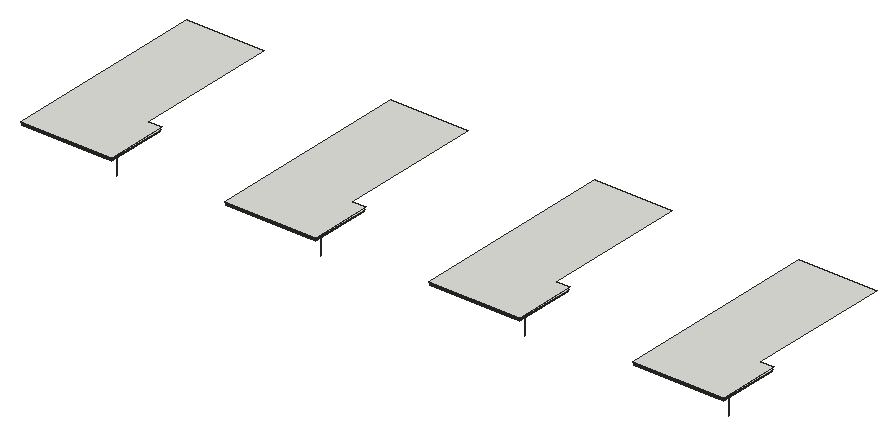
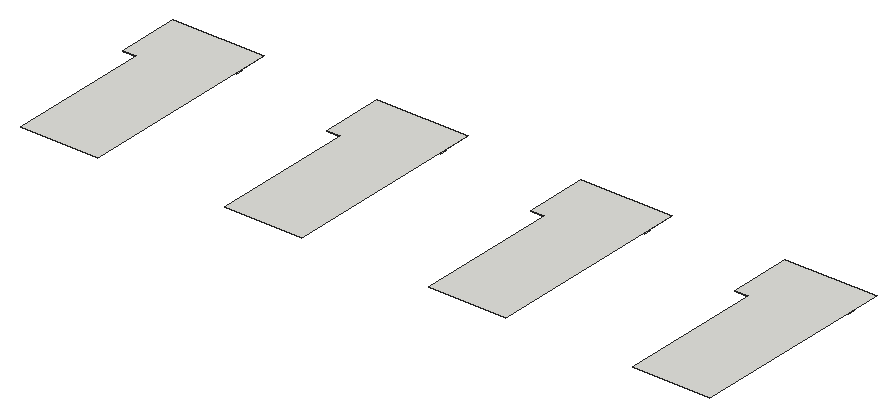
# SketchUp Ruby script. Lengths in inches.
U = 1.inch
M = Sketchup.active_model
def pt(a) = Geom::Point3d.new(a.map { |v| v * U })
def face(e, loops, mat)
  f = e.add_face(loops[0].map { |a| pt(a) })
  loops[1..].each { |l| e.add_face(l.map { |a| pt(a) }).erase! }
  f.material = f.back_material = mat if mat
  f
end
# faces: each face lists its corners as indices into pts; further lists are holes
def faces(e, pts, list, mat = nil) = list.each { |f| face(e, (f[0].is_a?(Array) ? f : [f]).map { |l| l.map { |i| pts[i] } }, mat) }
# xy, xz, yz: faces in a plane at the given z, y or x. An outline is a flat list of corners, or four numbers for a rectangle; further outlines are holes
def ring(l) = l.size == 4 ? [[l[0], l[1]], [l[2], l[1]], [l[2], l[3]], [l[0], l[3]]] : l.each_slice(2).to_a
def flat(e, list, mat, &to3) = list.each { |f| face(e, (f[0].is_a?(Array) ? f : [f]).map { |l| ring(l).map { |u, v| to3.(u, v) } }, mat) }
def xy(e, z, list, mat = nil) = flat(e, list, mat) { |x, y| [x, y, z] }
def xz(e, y, list, mat = nil) = flat(e, list, mat) { |x, z| [x, y, z] }
def yz(e, x, list, mat = nil) = flat(e, list, mat) { |y, z| [x, y, z] }
def lines(e, pts, list) = list.each { |a, b| e.add_line(pt(pts[a]), pt(pts[b])) }
# prism: a flat outline (further loops are holes) pulled along v
def prism(e, loops, v, mat = nil)
  f = face(e, loops, mat); d = Geom::Vector3d.new(v.map { |x| x * U })
  f.pushpull(f.normal.samedirection?(d) ? d.length : -d.length)
end
def box(e, o, s, mat = nil) = prism(e, [[o, [o[0] + s[0], o[1], o[2]], [o[0] + s[0], o[1] + s[1], o[2]], [o[0], o[1] + s[1], o[2]]]], [0, 0, s[2]], mat)
def at(x, y, z, deg = 0) = Geom::Transformation.translation(pt([x, y, z])) * Geom::Transformation.rotation(ORIGIN, Z_AXIS, deg.degrees)
def axes(o, x, y, z) = Geom::Transformation.new([*x, 0, *y, 0, *z, 0, *pt(o).to_a, 1])
def part(name) = M.definitions.add(name)
# library, detail: a bought-in or finely detailed component or shape, given as its bounding box
def library(name, o, s) = part(name).tap { |d| box(d.entities, o, s) }
def detail(e, o, s) = box(e.add_group.entities, o, s)
def put(e, d, t, mat = nil) = e.add_instance(d, t).tap { |i| i.material = mat if mat }
def group(e, t, mat = nil) = e.add_group.tap { |g| g.transformation = t; g.material = mat if mat }.entities
root = M.entities
M.materials.add("[0136_Charcoal]").color = [35, 35, 35]
M.materials.add("[Color M09]").color = [0, 0, 0]
M.materials.add("[Translucent Glass Gray]").color = [128, 128, 128]
M.materials["[Translucent Glass Gray]"].alpha = 0.5
xy(root,225.74,[[410.54,519.01,443.7,522.83],[1000.35,519.01,1033.52,522.83],[1590.16,519.01,1623.33,522.83],[2179.98,519.01,2213.14,522.83]])
xy(root,225.74,[[412.04,509.7,443.7,511.7],[445.2,509.7,475.37,511.7],[476.87,509.7,507.04,511.7],[1001.85,509.7,1033.52,511.7],[1035.02,509.7,1065.18,511.7],
  [1066.68,509.7,1096.85,511.7],[1591.66,509.7,1623.33,511.7],[1624.83,509.7,1655,511.7],[1656.5,509.7,1686.66,511.7],[2181.48,509.7,2213.14,511.7],
  [2214.64,509.7,2244.81,511.7],[2246.31,509.7,2276.48,511.7],[515.04,521.34,518.04,553.96],[1104.85,521.34,1107.85,553.96],[1694.66,521.34,1697.66,553.96],
  [2284.48,521.34,2287.48,553.96],[515.04,555.96,518.04,586.08],[1104.85,555.96,1107.85,586.08],[1694.66,555.96,1697.66,586.08],[2284.48,555.96,2287.48,586.08],
  [515.04,588.08,518.04,619.7],[1104.85,588.08,1107.85,619.7],[1694.66,588.08,1697.66,619.7],[2284.48,588.08,2287.48,619.7]],"[Color M09]")
xy(root,227.74,[[412.04,509.7,443.7,511.7],[445.2,509.7,475.37,511.7],[476.87,509.7,507.04,511.7],[1001.85,509.7,1033.52,511.7],[1035.02,509.7,1065.18,511.7],
  [1066.68,509.7,1096.85,511.7],[1591.66,509.7,1623.33,511.7],[1624.83,509.7,1655,511.7],[1656.5,509.7,1686.66,511.7],[2181.48,509.7,2213.14,511.7],
  [2214.64,509.7,2244.81,511.7],[2246.31,509.7,2276.48,511.7],[515.04,521.34,518.04,553.96],[1104.85,521.34,1107.85,553.96],[1694.66,521.34,1697.66,553.96],
  [2284.48,521.34,2287.48,553.96],[515.04,555.96,518.04,586.08],[1104.85,555.96,1107.85,586.08],[1694.66,555.96,1697.66,586.08],[2284.48,555.96,2287.48,586.08],
  [515.04,588.08,518.04,619.7],[1104.85,588.08,1107.85,619.7],[1694.66,588.08,1697.66,619.7],[2284.48,588.08,2287.48,619.7]],"[Color M09]")
xy(root,240.6,[[311.04,509.7,359.04,525.45],[900.85,509.7,948.85,525.45],[1490.66,509.7,1538.66,525.45],[2080.48,509.7,2128.48,525.45]])
xy(root,249.6875,[[443.7,509.7,445.2,511.7],[475.37,509.7,476.87,511.7],[1033.52,509.7,1035.02,511.7],[1065.18,509.7,1066.68,511.7],[1623.33,509.7,1624.83,511.7],
  [1655,509.7,1656.5,511.7],[2213.14,509.7,2214.64,511.7],[2244.81,509.7,2246.31,511.7],[410.54,511.7,443.7,522.83],[443.7,511.7,476.87,522.83],
  [476.87,511.7,508.54,519.01],[1000.35,511.7,1033.52,522.83],[1033.52,511.7,1066.68,522.83],[1066.68,511.7,1098.35,519.01],[1590.16,511.7,1623.33,522.83],
  [1623.33,511.7,1656.5,522.83],[1656.5,511.7,1688.16,519.01],[2179.98,511.7,2213.14,522.83],[2213.14,511.7,2246.31,522.83],[2246.31,511.7,2277.98,519.01]])
xy(root,249.6875,[[412.04,509.7,443.7,511.7],[445.2,509.7,475.37,511.7],[476.87,509.7,507.04,511.7],[1001.85,509.7,1033.52,511.7],[1035.02,509.7,1065.18,511.7],
  [1066.68,509.7,1096.85,511.7],[1591.66,509.7,1623.33,511.7],[1624.83,509.7,1655,511.7],[1656.5,509.7,1686.66,511.7],[2181.48,509.7,2213.14,511.7],
  [2214.64,509.7,2244.81,511.7],[2246.31,509.7,2276.48,511.7],[515.04,521.34,518.04,553.96],[1104.85,521.34,1107.85,553.96],[1694.66,521.34,1697.66,553.96],
  [2284.48,521.34,2287.48,553.96],[515.04,555.96,518.04,586.08],[1104.85,555.96,1107.85,586.08],[1694.66,555.96,1697.66,586.08],[2284.48,555.96,2287.48,586.08],
  [515.04,588.08,518.04,619.7],[1104.85,588.08,1107.85,619.7],[1694.66,588.08,1697.66,619.7],[2284.48,588.08,2287.48,619.7]],"[Color M09]")
xy(root,251.6875,[[544.21,449.7,557.59,468.65],[1134.02,449.7,1147.4,468.65],[1723.83,449.7,1737.22,468.65],[2313.65,449.7,2327.03,468.65],[410.04,509.7,509.04,511.7],
  [999.85,509.7,1098.85,511.7],[1589.66,509.7,1688.66,511.7],[2179.48,509.7,2278.48,511.7],[503.73,519.34,515.04,555.96],[515.04,519.34,518.04,621.7],
  [1093.54,519.34,1104.85,555.96],[1104.85,519.34,1107.85,621.7],[1683.35,519.34,1694.66,555.96],[1694.66,519.34,1697.66,621.7],[2273.16,519.34,2284.48,555.96],
  [2284.48,519.34,2287.48,621.7],[503.73,555.96,515.04,588.08],[1093.54,555.96,1104.85,588.08],[1683.35,555.96,1694.66,588.08],[2273.16,555.96,2284.48,588.08],
  [503.73,588.08,515.04,621.7],[1093.54,588.08,1104.85,621.7],[1683.35,588.08,1694.66,621.7],[2273.16,588.08,2284.48,621.7]])
xy(root,251.6875,[[302.04,449.7,544.21,509.7],[891.85,449.7,1134.02,509.7],[1481.66,449.7,1723.83,509.7],[2071.48,449.7,2313.65,509.7],[544.21,468.65,544.21,509.7,518.04,509.7,518.04,621.7,557.59,621.7,557.59,468.65],
  [1134.02,468.65,1134.02,509.7,1107.85,509.7,1107.85,621.7,1147.4,621.7,1147.4,468.65],[1723.83,468.65,1723.83,509.7,1697.66,509.7,1697.66,621.7,1737.22,621.7,1737.22,468.65],[2313.65,468.65,2313.65,509.7,2287.48,509.7,2287.48,621.7,2327.03,621.7,2327.03,468.65]],"[0136_Charcoal]")
xy(root,255.07,[[297.83,449.7,557.59,450.7],[887.64,449.7,1147.4,450.7],[1477.46,449.7,1737.22,450.7],[2067.27,449.7,2327.03,450.7],[556.59,450.7,557.59,624.51],
  [1146.4,450.7,1147.4,624.51],[1736.22,450.7,1737.22,624.51],[2326.03,450.7,2327.03,624.51]],"[0136_Charcoal]")
xy(root,256.21,[[296.69,449.7,557.59,450.7],[886.5,449.7,1147.4,450.7],[1476.32,449.7,1737.22,450.7],[2066.13,449.7,2327.03,450.7],[556.59,450.7,557.59,625.64],
  [1146.4,450.7,1147.4,625.64],[1736.22,450.7,1737.22,625.64],[2326.03,450.7,2327.03,625.64]])
xy(root,259.6875,[[293.22,449.7,557.59,449.7,557.59,629.7,518.04,629.7,518.04,1049.7,293.22,1049.7],[883.03,449.7,1147.4,449.7,1147.4,629.7,1107.85,629.7,1107.85,1049.7,883.03,1049.7],[1472.84,449.7,1737.22,449.7,1737.22,629.7,1697.66,629.7,1697.66,1049.7,1472.84,1049.7],[2062.65,449.7,2327.03,449.7,2327.03,629.7,2287.48,629.7,2287.48,1049.7,2062.65,1049.7]])
xz(root,510.7,[[412.04,227.74,443.7,249.6875],[445.2,227.74,475.37,249.6875],[476.87,227.74,507.04,249.6875],[1001.85,227.74,1033.52,249.6875],[1035.02,227.74,1065.18,249.6875],
  [1066.68,227.74,1096.85,249.6875],[1591.66,227.74,1623.33,249.6875],[1624.83,227.74,1655,249.6875],[1656.5,227.74,1686.66,249.6875],[2181.48,227.74,2213.14,249.6875],
  [2214.64,227.74,2244.81,249.6875],[2246.31,227.74,2276.48,249.6875]],"[Translucent Glass Gray]")
xz(root,511.7,[[412.04,225.74,443.7,227.74],[445.2,225.74,475.37,227.61],[476.87,225.74,507.04,227.74],[507.04,225.74,508.54,249.6875],[1001.85,225.74,1033.52,227.74],
  [1035.02,225.74,1065.18,227.61],[1066.68,225.74,1096.85,227.74],[1096.85,225.74,1098.35,249.6875],[1591.66,225.74,1623.33,227.74],[1624.83,225.74,1655,227.61],
  [1656.5,225.74,1686.66,227.74],[1686.66,225.74,1688.16,249.6875],[2181.48,225.74,2213.14,227.74],[2214.64,225.74,2244.81,227.61],[2246.31,225.74,2276.48,227.74],
  [2276.48,225.74,2277.98,249.6875],[410.54,227.74,412.04,249.6875],[443.7,227.74,445.2,231.3],[475.37,227.74,476.87,249.6875],[1000.35,227.74,1001.85,249.6875],
  [1033.52,227.74,1035.02,231.3],[1065.18,227.74,1066.68,249.6875],[1590.16,227.74,1591.66,249.6875],[1623.33,227.74,1624.83,231.3],[1655,227.74,1656.5,249.6875],
  [2179.98,227.74,2181.48,249.6875],[2213.14,227.74,2214.64,231.3],[2244.81,227.74,2246.31,249.6875],[443.7,231.3,445.2,249.6875],[1033.52,231.3,1035.02,249.6875],
  [1623.33,231.3,1624.83,249.6875],[2213.14,231.3,2214.64,249.6875]])
xz(root,519.01,[[410.54,225.74,443.7,227.74],[476.87,225.74,508.54,249.6875],[1000.35,225.74,1033.52,227.74],[1066.68,225.74,1098.35,249.6875],[1590.16,225.74,1623.33,227.74],
  [1656.5,225.74,1688.16,249.6875],[2179.98,225.74,2213.14,227.74],[2246.31,225.74,2277.98,249.6875]])
xz(root,519.34,[[503.73,224.74,515.04,251.6875],[1093.54,224.74,1104.85,251.6875],[1683.35,224.74,1694.66,251.6875],[2273.16,224.74,2284.48,251.6875]])
xz(root,521.34,[[515.04,227.74,518.04,249.6875],[1104.85,227.74,1107.85,249.6875],[1694.66,227.74,1697.66,249.6875],[2284.48,227.74,2287.48,249.6875]],"[Color M09]")
xz(root,522.83,[[410.54,225.74,443.7,249.6875],[1000.35,225.74,1033.52,249.6875],[1590.16,225.74,1623.33,249.6875],[2179.98,225.74,2213.14,249.6875],[443.7,227.74,476.87,249.6875],
  [1033.52,227.74,1066.68,249.6875],[1623.33,227.74,1656.5,249.6875],[2213.14,227.74,2246.31,249.6875]])
xz(root,553.96,[[515.04,227.74,518.04,249.6875],[1104.85,227.74,1107.85,249.6875],[1694.66,227.74,1697.66,249.6875],[2284.48,227.74,2287.48,249.6875]],"[Color M09]")
xz(root,555.96,[[515.04,227.74,518.04,249.6875],[1104.85,227.74,1107.85,249.6875],[1694.66,227.74,1697.66,249.6875],[2284.48,227.74,2287.48,249.6875]],"[Color M09]")
xz(root,586.08,[[515.04,227.74,518.04,249.6875],[1104.85,227.74,1107.85,249.6875],[1694.66,227.74,1697.66,249.6875],[2284.48,227.74,2287.48,249.6875]],"[Color M09]")
xz(root,588.08,[[515.04,227.74,518.04,249.6875],[1104.85,227.74,1107.85,249.6875],[1694.66,227.74,1697.66,249.6875],[2284.48,227.74,2287.48,249.6875]],"[Color M09]")
xz(root,619.7,[[515.04,227.74,518.04,249.6875],[1104.85,227.74,1107.85,249.6875],[1694.66,227.74,1697.66,249.6875],[2284.48,227.74,2287.48,249.6875]],"[Color M09]")
xz(root,621.7,[[503.73,224.74,515.04,251.6875],[1093.54,224.74,1104.85,251.6875],[1683.35,224.74,1694.66,251.6875],[2273.16,224.74,2284.48,251.6875]])
yz(root,410.54,[[519.01,225.74,522.83,225.74,522.83,249.6875,511.7,249.6875,511.7,227.74,519.01,227.74]])
yz(root,412.04,[[509.7,227.74,511.7,249.6875]],"[Color M09]")
yz(root,443.7,[[519.01,225.74,522.83,227.74]])
yz(root,443.7,[[509.7,227.74,511.7,249.6875]],"[Color M09]")
yz(root,445.2,[[509.7,227.74,511.7,231.3],[509.7,231.3,511.7,249.6875]],"[Color M09]")
yz(root,475.37,[[509.7,227.74,511.7,249.6875]],"[Color M09]")
yz(root,476.87,[[509.7,227.74,511.7,249.6875]],"[Color M09]")
yz(root,503.73,[[519.34,224.74,555.96,251.6875],[555.96,224.74,588.08,251.6875],[588.08,224.74,621.7,251.6875]])
yz(root,507.04,[[509.7,227.74,511.7,249.6875]],"[Color M09]")
yz(root,508.54,[[511.7,225.74,519.01,249.6875]])
yz(root,515.04,[[519.34,168.6875,521.34,224.74],[519.34,224.74,519.34,251.6875,522.34,251.6875,522.34,249.6875,521.34,249.6875,521.34,227.74,522.34,227.74,522.34,225.74,521.34,225.74,521.34,224.74],[553.96,224.74,553.96,225.74,552.96,225.74,552.96,227.74,553.96,227.74,553.96,249.6875,552.96,249.6875,552.96,251.6875,555.96,251.6875,555.96,224.74],[586.08,224.74,586.08,225.74,585.08,225.74,585.08,227.74,586.08,227.74,586.08,249.6875,585.08,249.6875,585.08,251.6875,588.08,251.6875,588.08,224.74],[619.7,224.74,619.7,225.74,588.08,225.74,588.08,227.74,621.7,227.74,621.7,224.74],
  [522.34,225.74,552.96,227.74],[555.96,225.74,585.08,227.74],[619.7,227.74,621.7,248.6875],[619.7,248.6875,619.7,249.6875,588.08,249.6875,588.08,251.6875,621.7,251.6875,621.7,248.6875],[522.34,249.6875,552.96,251.6875],
  [555.96,249.6875,585.08,251.6875]])
yz(root,516.54,[[521.34,227.74,553.96,249.6875],[588.08,227.74,619.7,249.6875]],"[Translucent Glass Gray]")
yz(root,1000.35,[[519.01,225.74,522.83,225.74,522.83,249.6875,511.7,249.6875,511.7,227.74,519.01,227.74]])
yz(root,1001.85,[[509.7,227.74,511.7,249.6875]],"[Color M09]")
yz(root,1033.52,[[519.01,225.74,522.83,227.74]])
yz(root,1033.52,[[509.7,227.74,511.7,249.6875]],"[Color M09]")
yz(root,1035.02,[[509.7,227.74,511.7,231.3],[509.7,231.3,511.7,249.6875]],"[Color M09]")
yz(root,1065.18,[[509.7,227.74,511.7,249.6875]],"[Color M09]")
yz(root,1066.68,[[509.7,227.74,511.7,249.6875]],"[Color M09]")
yz(root,1093.54,[[519.34,224.74,555.96,251.6875],[555.96,224.74,588.08,251.6875],[588.08,224.74,621.7,251.6875]])
yz(root,1096.85,[[509.7,227.74,511.7,249.6875]],"[Color M09]")
yz(root,1098.35,[[511.7,225.74,519.01,249.6875]])
yz(root,1104.85,[[519.34,168.6875,521.34,224.74],[519.34,224.74,519.34,251.6875,522.34,251.6875,522.34,249.6875,521.34,249.6875,521.34,227.74,522.34,227.74,522.34,225.74,521.34,225.74,521.34,224.74],[553.96,224.74,553.96,225.74,552.96,225.74,552.96,227.74,553.96,227.74,553.96,249.6875,552.96,249.6875,552.96,251.6875,555.96,251.6875,555.96,224.74],[586.08,224.74,586.08,225.74,585.08,225.74,585.08,227.74,586.08,227.74,586.08,249.6875,585.08,249.6875,585.08,251.6875,588.08,251.6875,588.08,224.74],[619.7,224.74,619.7,225.74,588.08,225.74,588.08,227.74,621.7,227.74,621.7,224.74],
  [522.34,225.74,552.96,227.74],[555.96,225.74,585.08,227.74],[619.7,227.74,621.7,248.6875],[619.7,248.6875,619.7,249.6875,588.08,249.6875,588.08,251.6875,621.7,251.6875,621.7,248.6875],[522.34,249.6875,552.96,251.6875],
  [555.96,249.6875,585.08,251.6875]])
yz(root,1106.35,[[521.34,227.74,553.96,249.6875],[588.08,227.74,619.7,249.6875]],"[Translucent Glass Gray]")
yz(root,1590.16,[[519.01,225.74,522.83,225.74,522.83,249.6875,511.7,249.6875,511.7,227.74,519.01,227.74]])
yz(root,1591.66,[[509.7,227.74,511.7,249.6875]],"[Color M09]")
yz(root,1623.33,[[519.01,225.74,522.83,227.74]])
yz(root,1623.33,[[509.7,227.74,511.7,249.6875]],"[Color M09]")
yz(root,1624.83,[[509.7,227.74,511.7,231.3],[509.7,231.3,511.7,249.6875]],"[Color M09]")
yz(root,1655,[[509.7,227.74,511.7,249.6875]],"[Color M09]")
yz(root,1656.5,[[509.7,227.74,511.7,249.6875]],"[Color M09]")
yz(root,1683.35,[[519.34,224.74,555.96,251.6875],[555.96,224.74,588.08,251.6875],[588.08,224.74,621.7,251.6875]])
yz(root,1686.66,[[509.7,227.74,511.7,249.6875]],"[Color M09]")
yz(root,1688.16,[[511.7,225.74,519.01,249.6875]])
yz(root,1694.66,[[519.34,168.6875,521.34,224.74],[519.34,224.74,519.34,251.6875,522.34,251.6875,522.34,249.6875,521.34,249.6875,521.34,227.74,522.34,227.74,522.34,225.74,521.34,225.74,521.34,224.74],[553.96,224.74,553.96,225.74,552.96,225.74,552.96,227.74,553.96,227.74,553.96,249.6875,552.96,249.6875,552.96,251.6875,555.96,251.6875,555.96,224.74],[586.08,224.74,586.08,225.74,585.08,225.74,585.08,227.74,586.08,227.74,586.08,249.6875,585.08,249.6875,585.08,251.6875,588.08,251.6875,588.08,224.74],[619.7,224.74,619.7,225.74,588.08,225.74,588.08,227.74,621.7,227.74,621.7,224.74],
  [522.34,225.74,552.96,227.74],[555.96,225.74,585.08,227.74],[619.7,227.74,621.7,248.6875],[619.7,248.6875,619.7,249.6875,588.08,249.6875,588.08,251.6875,621.7,251.6875,621.7,248.6875],[522.34,249.6875,552.96,251.6875],
  [555.96,249.6875,585.08,251.6875]])
yz(root,1696.16,[[521.34,227.74,553.96,249.6875],[588.08,227.74,619.7,249.6875]],"[Translucent Glass Gray]")
yz(root,2179.98,[[519.01,225.74,522.83,225.74,522.83,249.6875,511.7,249.6875,511.7,227.74,519.01,227.74]])
yz(root,2181.48,[[509.7,227.74,511.7,249.6875]],"[Color M09]")
yz(root,2213.14,[[519.01,225.74,522.83,227.74]])
yz(root,2213.14,[[509.7,227.74,511.7,249.6875]],"[Color M09]")
yz(root,2214.64,[[509.7,227.74,511.7,231.3],[509.7,231.3,511.7,249.6875]],"[Color M09]")
yz(root,2244.81,[[509.7,227.74,511.7,249.6875]],"[Color M09]")
yz(root,2246.31,[[509.7,227.74,511.7,249.6875]],"[Color M09]")
yz(root,2273.16,[[519.34,224.74,555.96,251.6875],[555.96,224.74,588.08,251.6875],[588.08,224.74,621.7,251.6875]])
yz(root,2276.48,[[509.7,227.74,511.7,249.6875]],"[Color M09]")
yz(root,2277.98,[[511.7,225.74,519.01,249.6875]])
yz(root,2284.48,[[519.34,168.6875,521.34,224.74],[519.34,224.74,519.34,251.6875,522.34,251.6875,522.34,249.6875,521.34,249.6875,521.34,227.74,522.34,227.74,522.34,225.74,521.34,225.74,521.34,224.74],[553.96,224.74,553.96,225.74,552.96,225.74,552.96,227.74,553.96,227.74,553.96,249.6875,552.96,249.6875,552.96,251.6875,555.96,251.6875,555.96,224.74],[586.08,224.74,586.08,225.74,585.08,225.74,585.08,227.74,586.08,227.74,586.08,249.6875,585.08,249.6875,585.08,251.6875,588.08,251.6875,588.08,224.74],[619.7,224.74,619.7,225.74,588.08,225.74,588.08,227.74,621.7,227.74,621.7,224.74],
  [522.34,225.74,552.96,227.74],[555.96,225.74,585.08,227.74],[619.7,227.74,621.7,248.6875],[619.7,248.6875,619.7,249.6875,588.08,249.6875,588.08,251.6875,621.7,251.6875,621.7,248.6875],[522.34,249.6875,552.96,251.6875],
  [555.96,249.6875,585.08,251.6875]])
yz(root,2285.98,[[521.34,227.74,553.96,249.6875],[588.08,227.74,619.7,249.6875]],"[Translucent Glass Gray]")
p = [[476.87,519.01,227.74],[476.87,522.83,227.74],[1066.68,519.01,227.74],[1066.68,522.83,227.74],[1656.5,519.01,227.74],[1656.5,522.83,227.74],
  [2246.31,519.01,227.74],[2246.31,522.83,227.74]]
lines(root,p,[[0,1],[2,3],[4,5],[6,7]])
